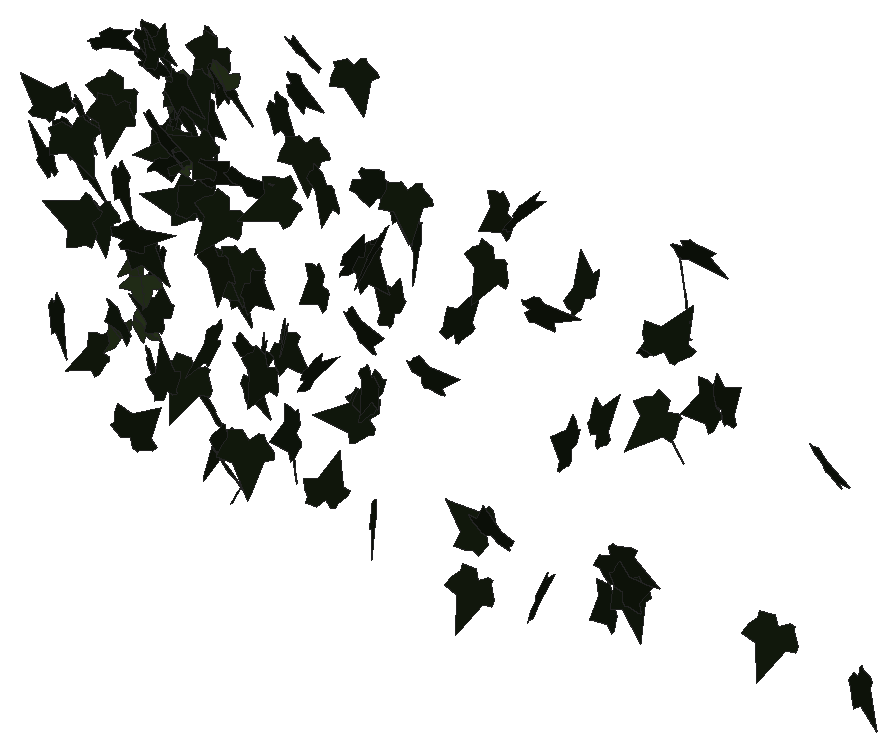
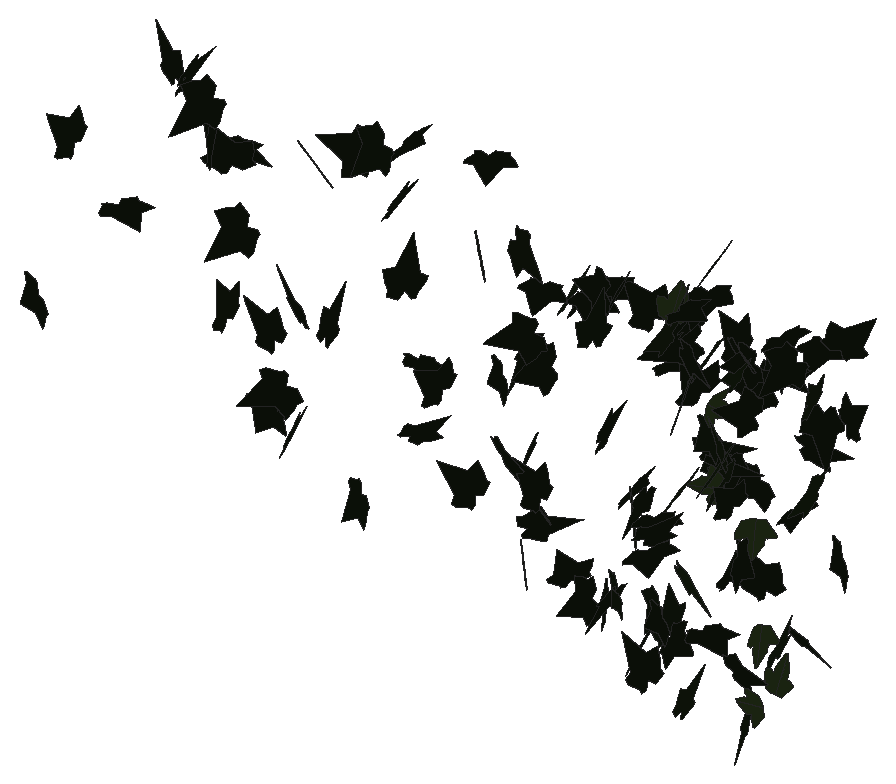
# SketchUp Ruby script. Lengths in inches.
U = 1.inch
M = Sketchup.active_model
def pt(a) = Geom::Point3d.new(a.map { |v| v * U })
def face(e, loops, mat)
  f = e.add_face(loops[0].map { |a| pt(a) })
  loops[1..].each { |l| e.add_face(l.map { |a| pt(a) }).erase! }
  f.material = f.back_material = mat if mat
  f
end
# faces: each face lists its corners as indices into pts; further lists are holes
def faces(e, pts, list, mat = nil) = list.each { |f| face(e, (f[0].is_a?(Array) ? f : [f]).map { |l| l.map { |i| pts[i] } }, mat) }
# xy, xz, yz: faces in a plane at the given z, y or x. An outline is a flat list of corners, or four numbers for a rectangle; further outlines are holes
def ring(l) = l.size == 4 ? [[l[0], l[1]], [l[2], l[1]], [l[2], l[3]], [l[0], l[3]]] : l.each_slice(2).to_a
def flat(e, list, mat, &to3) = list.each { |f| face(e, (f[0].is_a?(Array) ? f : [f]).map { |l| ring(l).map { |u, v| to3.(u, v) } }, mat) }
def xy(e, z, list, mat = nil) = flat(e, list, mat) { |x, y| [x, y, z] }
def xz(e, y, list, mat = nil) = flat(e, list, mat) { |x, z| [x, y, z] }
def yz(e, x, list, mat = nil) = flat(e, list, mat) { |y, z| [x, y, z] }
def lines(e, pts, list) = list.each { |a, b| e.add_line(pt(pts[a]), pt(pts[b])) }
# prism: a flat outline (further loops are holes) pulled along v
def prism(e, loops, v, mat = nil)
  f = face(e, loops, mat); d = Geom::Vector3d.new(v.map { |x| x * U })
  f.pushpull(f.normal.samedirection?(d) ? d.length : -d.length)
end
def box(e, o, s, mat = nil) = prism(e, [[o, [o[0] + s[0], o[1], o[2]], [o[0] + s[0], o[1] + s[1], o[2]], [o[0], o[1] + s[1], o[2]]]], [0, 0, s[2]], mat)
def at(x, y, z, deg = 0) = Geom::Transformation.translation(pt([x, y, z])) * Geom::Transformation.rotation(ORIGIN, Z_AXIS, deg.degrees)
def axes(o, x, y, z) = Geom::Transformation.new([*x, 0, *y, 0, *z, 0, *pt(o).to_a, 1])
def part(name) = M.definitions.add(name)
# library, detail: a bought-in or finely detailed component or shape, given as its bounding box
def library(name, o, s) = part(name).tap { |d| box(d.entities, o, s) }
def detail(e, o, s) = box(e.add_group.entities, o, s)
def put(e, d, t, mat = nil) = e.add_instance(d, t).tap { |i| i.material = mat if mat }
def group(e, t, mat = nil) = e.add_group.tap { |g| g.transformation = t; g.material = mat if mat }.entities
root = M.entities
M.materials.add("efeu1").color = [18, 25, 13]
M.materials.add("efeu2").color = [43, 57, 29]
c1 = part("ivyleaf_9")
p = [[1.54,2.16,1.25],[1.36,2.04,1.19],[-0.21,0.99,0.68],[-0.71,1.11,0.82],[-0.85,0.86,0.67],[-0.8,0.17,0.21],
  [-0.9,-0.01,0.1],[-0.67,-0.16,-0.02],[-0.08,-0.08,-0.05],[-0.03,-0.6,-0.4],[0.65,-0.88,-0.66],[0.83,-0.6,-0.49],
  [1.29,-0.42,-0.43],[1.8125,-0.07,-0.26],[1.21,0.44,0.15]]
faces(c1.entities,p,[[0,1,2,3,4,5,6,7,8,9,10,11,12,13,14]],"efeu1")
c2 = part("ivyleaf_10")
p = [[0,0.5,-0.03],[-0.0625,2.02,-0.43],[-0.19,2.01,-0.46],[-0.54,1.05,-0.29],[-0.52,0.625,-0.18],[-0.83,0.76,-0.28],
  [-1.16,0.64,-0.33],[-1.15,0.33,-0.24],[-0.77,-0.39,0.02],[-0.3,-0.51,0.16],[0.04,-0.48,0.23],[-0.02,2.01,-0.4375],
  [-0.06,2.01,-0.43],[0.04,-0.49,0.23],[0.67,-0.49,0.14],[1.38,0.36,-0.2],[1.375,0.51,-0.24],[0.81,0.65,-0.19],
  [0.62,0.59,-0.15],[0.6,1.09,-0.28],[0.5,1.23,-0.31]]
faces(c2.entities,p,[[0,1,2,3,4,5,6,7,8,9,10],[11,12,0,13,14,15,16,17,18,19,20]],"efeu2")
put(root,c1,axes([622.18,119.2,263.21],[1.07027,-0.87994,-0.07632],[-0.0577,0.04999,-1.38556],[0.88136,1.07182,0.00197]))
put(root,c2,axes([623.27,124.4375,252.77],[-0.24136,-1.16635,-0.4298],[0.08796,0.4207,-1.19106],[1.2399,-0.25688,0.00083]))
put(root,c1,axes([623.84,113.15,265.97],[0.21287,-0.39615,1.24207],[-0.67814,1.04122,0.44831],[-1.11347,-0.70987,-0.03558]))
put(root,c1,axes([623.82,116.15,267.9375],[0.91937,0.46952,-1.02129],[-0.91999,-0.44374,-1.03219],[-0.64582,1.30052,0.01652]))
put(root,c2,axes([623.56,122.17,247.09],[-0.30293,-0.92854,-0.79827],[-0.11742,-0.79652,0.97106],[-1.21887,0.30751,0.10485]))
put(root,c2,axes([623.04,125.3,246.88],[-0.31561,0.08385,-1.18043],[1.06121,-0.52059,-0.32072],[-0.5237,-1.10544,0.0615]))
put(root,c1,axes([623.75,119.875,274.29],[0.96359,0.79758,0.36569],[0.28178,0.23309,-1.25086],[-0.83094,1.00394,-0.00011]))
put(root,c1,axes([625.05,112.375,271.84],[0.34068,0.08173,1.27704],[-1.27575,0.12473,0.33236],[-0.09978,-1.3158,0.11083]))
put(root,c1,axes([624.23,121.375,249.1875],[0.80971,-0.82826,-0.57852],[0.44902,-0.36912,1.15692],[-0.90503,-0.92416,0.05641]))
put(root,c1,axes([624.83,124.15,244.65],[0.77824,-0.30414,-0.90228],[-0.84618,0.31337,-0.83549],[0.43656,1.14959,-0.01096]))
put(root,c1,axes([625.83,124.41,248.55],[-0.49007,0.3241,1.15418],[-0.93577,0.67596,-0.58715],[-0.74933,-1.05611,-0.02161]))
put(root,c1,axes([625.77,117.2,248.65],[-1.16585,0.35783,0.27903],[-0.26928,0.07359,-1.21949],[-0.36522,-1.19651,0.00844]))
put(root,c1,axes([624.35,116.86,269.05],[0.277,-0.84104,1.03036],[0.28803,-0.98956,-0.88517],[1.29847,0.39892,-0.02345]))
put(root,c1,axes([624.78,118.23,260.3],[0.0021,-1.203,-0.29037],[0.00436,0.29038,-1.20299],[1.23754,0.00102,0.00473]))
put(root,c1,axes([624.51,113.15,253.97],[-0.26944,-0.07175,-1.46481],[1.46634,-0.03975,-0.26777],[-0.02617,-1.48886,0.07774]))
put(root,c1,axes([625.69,124.93,263.3],[-0.31911,-0.34503,1.1605],[0.75283,0.88335,0.46964],[-0.94818,0.81748,-0.01768]))
put(root,c1,axes([624.77,123.65,270.93],[0.86711,-0.31452,0.89042],[0.83413,-0.31165,-0.92237],[0.44273,1.20316,-0.00615]))
put(root,c1,axes([625.96,125.93,267.32],[0.90464,-1.06864,-0.39949],[-0.25391,0.30847,-1.40012],[1.11226,0.93958,0.0053]))
put(root,c1,axes([627.81,113.16,262.51],[-0.88339,-0.44861,-1.11531],[-0.97594,-0.54051,0.99041],[-0.70192,1.31611,0.02659]))
put(root,c1,axes([627,117.99,271.59],[-1.15565,-0.89341,0.10894],[-0.06996,-0.0876,-1.46049],[0.89731,-1.15747,0.02644]))
put(root,c1,axes([625.91,122.21,274.46],[0.15475,0.02861,-1.2753],[1.15452,0.54319,0.15228],[0.54249,-1.16417,0.03971]))
put(root,c1,axes([628.12,121.07,273.8],[-0.28165,0.51474,1.17737],[-0.65843,0.97725,-0.58476],[-1.10347,-0.7145,0.04841]))
put(root,c1,axes([626.48,122.77,273.85],[0.77343,-0.98251,0.29118],[0.17618,-0.23187,-1.2504],[1.00949,0.79323,-0.00486]))
put(root,c1,axes([627.22,124.08,266.52],[-0.18666,0.93539,0.88445],[0.18438,-0.86506,0.95379],[1.27405,0.26223,-0.00846]))
put(root,c1,axes([627.3,111.75,271.08],[-0.23408,-0.97827,-1.00749],[0.26411,0.97249,-1.00565],[1.37923,-0.35225,0.02158]))
put(root,c1,axes([628.34,124.27,268.51],[-0.60417,0.68238,-1.01169],[-0.7456,0.68726,0.90882],[0.96605,0.95719,0.06871]))
put(root,c1,axes([627.82,122.83,265.22],[1.01108,-0.07908,-0.8091],[-0.75922,0.36981,-0.98489],[0.29066,1.24104,0.24192]))
put(root,c1,axes([628.98,122.97,264.77],[-0.92686,-0.02912,0.90525],[-0.89854,-0.13313,-0.92428],[0.11376,-1.28873,0.07503]))
put(root,c1,axes([628.17,121.08,256.2],[-0.35432,0.30629,-1.39728],[1.10967,-0.84953,-0.46761],[-0.90268,-1.16456,-0.02638]))
put(root,c1,axes([628.85,121.47,264.74],[0.40682,1.19247,-0.27089],[-0.08824,-0.25611,-1.25996],[-1.21967,0.41628,0.00081]))
put(root,c2,axes([628.59,123.68,270.375],[-0.11528,-0.76405,1.00801],[0.36573,-0.98909,-0.70788],[1.21083,0.22601,0.30978]))
put(root,c2,axes([628.01,123.84,263.55],[0.15172,-0.20456,1.22546],[1.15878,0.46861,-0.06525],[-0.44814,1.14245,0.24618]))
put(root,c1,axes([629.08,114.7,272.33],[-0.3971,-1.2906,-0.0785],[0.02506,0.07442,-1.35031],[1.29274,-0.39788,0.00207]))
put(root,c2,axes([629.93,116.92,256.45],[-0.99413,-0.79052,-0.06912],[0.05445,0.04258,-1.27013],[0.79167,-0.99562,0.00056]))
put(root,c1,axes([631.32,123.69,274.27],[-0.23925,-0.04646,-1.29065],[-1.27695,-0.18787,0.24347],[-0.19322,1.29913,-0.01094]))
put(root,c1,axes([630.01,116.37,260.27],[-0.13631,-0.21723,-1.44326],[1.28299,0.6732,-0.2225],[0.69579,-1.28389,0.12753]))
put(root,c1,axes([631.76,123.4375,242.82],[0.69343,-1.07414,0.27797],[-0.14309,0.23848,1.2785],[-1.10026,-0.70798,0.00892]))
put(root,c1,axes([632.78,119.19,263.15],[-0.60952,-0.00036,1.19221],[-1.18995,-0.08215,-0.60839],[0.07331,-1.33646,0.03708]))
put(root,c1,axes([631.26,126.67,252.28],[-0.18518,-0.11555,-1.22632],[1.21137,0.20757,-0.20248],[0.22314,-1.22273,0.08152]))
put(root,c1,axes([632.2,120.18,247.92],[-1.05369,-1.03255,-0.1616],[0.11127,0.11735,-1.47526],[1.03918,-1.05953,-0.0059]))
put(root,c1,axes([631.47,120.54,272.29],[0.80313,-1.25451,-0.12099],[-0.06212,0.10389,-1.48957],[1.2588,0.80552,0.00369]))
put(root,c1,axes([631.42,112.3,268.39],[-0.2568,-0.10479,-1.39468],[1.3967,0.05486,-0.26129],[0.07306,-1.41706,0.09302]))
put(root,c1,axes([632.64,121.67,269.87],[0.68175,-0.29692,-1.08173],[-0.92173,0.57315,-0.73824],[0.6393,1.14299,0.08918]))
put(root,c1,axes([632.33,115.8,270.74],[0.22031,-0.5165,1.38292],[0.83994,-1.10599,-0.54688],[1.21398,0.85895,0.12741]))
put(root,c1,axes([633.59,121.35,276.01],[-0.65952,-1.09232,0.3337],[-0.17864,-0.28195,-1.27596],[1.1281,-0.68324,-0.00696]))
put(root,c1,axes([634.04,114.76,249.52],[-0.44697,-0.88498,0.81564],[0.35961,0.73212,0.99142],[-1.14854,0.57363,-0.007]))
put(root,c1,axes([632.85,126.42,246.47],[-0.0673,-0.27756,1.4356],[1.06227,-0.99684,-0.14293],[1.00478,1.03528,0.24727]))
put(root,c1,axes([634.93,119.57,251.89],[-1.22281,0.66405,-0.36378],[0.30845,-0.19418,-1.3913],[-0.69149,-1.26091,0.02268]))
put(root,c1,axes([633.47,110.47,264.24],[0.59624,-0.00277,1.21045],[1.20694,0.10396,-0.59428],[-0.09204,1.34531,0.04842]))
put(root,c1,axes([633.86,110.71,247.08],[-0.49127,0.04059,1.4223],[1.23333,-0.7382,0.44707],[0.70956,1.31123,0.20766]))
put(root,c1,axes([634.4,117.12,275.39],[-0.22894,-1.17344,-0.9063],[0.14169,0.89553,-1.19529],[1.4759,-0.268,-0.02584]))
put(root,c1,axes([635.96,122.51,255.85],[-0.79796,-1.07819,-0.15225],[-0.05484,-0.14873,1.34063],[-1.08751,0.79862,0.04412]))
put(root,c1,axes([635.07,122.62,257.91],[-0.496,-1.10169,-0.50895],[0.25937,0.44088,-1.20712],[1.18553,-0.55738,0.05116]))
put(root,c2,axes([635.63,119.71,274.39],[-0.96165,-0.72892,-0.38434],[-0.29624,-0.24538,1.20658],[-0.76895,1.00612,0.01582]))
put(root,c1,axes([634.76,121.05,273.53],[1.01452,-0.84116,0.1064],[0.09072,-0.05727,-1.31781],[0.84299,1.01848,0.01377]))
put(root,c1,axes([634.92,119.95,258.86],[0.20491,-1.34864,0.64485],[0.13917,-0.63084,-1.36357],[1.48839,0.24466,0.03873]))
put(root,c1,axes([635.2,119.86,274.66],[0.17078,-0.82121,0.94718],[0.14708,-0.9362,-0.83821],[1.24495,0.22326,-0.03091]))
put(root,c1,axes([635.53,113.87,277.01],[0.88927,-0.64732,-0.83166],[-0.48519,0.71453,-1.07495],[0.93556,0.98585,0.23303]))
put(root,c1,axes([635.87,122.6,247.44],[0.79596,-0.77627,-0.72363],[-0.52901,0.49392,-1.11174],[0.91999,0.95563,-0.0132]))
put(root,c1,axes([636.26,115.63,265.55],[-0.5266,-0.48738,1.32358],[0.94978,0.92196,0.71737],[-1.04275,1.08589,-0.01501]))
put(root,c1,axes([636.92,118.26,244.9],[-0.17471,0.28734,-1.27841],[0.78194,-1.01203,-0.33433],[-1.0514,-0.8004,-0.03621]))
put(root,c1,axes([637.51,115.73,270.51],[-0.04019,-1.39427,-0.33401],[0.01694,-0.33458,1.39461],[-1.43362,0.03513,0.02584]))
put(root,c1,axes([638.36,123.11,250.39],[-0.08043,0.44334,1.26449],[-0.12729,1.25851,-0.44934],[-1.3339,-0.14683,-0.03337]))
put(root,c1,axes([637.8125,126.75,274.55],[1.17749,-0.62437,0.12941],[-0.10996,0.06886,1.33276],[-0.62809,-1.18258,0.00928]))
put(root,c1,axes([638.11,120.04,257.71],[0.43166,-0.46621,-1.10809],[-0.67274,0.88207,-0.63318],[0.99631,0.79759,0.05255]))
put(root,c1,axes([637.36,115.35,269.32],[1.17512,0.32103,0.82368],[0.80095,0.19327,-1.21801],[-0.37416,1.42197,-0.02041]))
put(root,c1,axes([638.19,123.79,250.8],[0.60817,-0.66893,-0.96136],[-0.45712,0.86175,-0.88881],[1.0783,0.74261,0.16543]))
put(root,c1,axes([639.64,115.19,266.71],[-0.79558,-1.14656,0.49012],[-0.22827,-0.43763,-1.39432],[1.22585,-0.82562,0.05844]))
put(root,c1,axes([638.94,115.86,244.03],[1.18805,-0.46251,-0.71038],[0.66346,-0.25392,1.2749],[-0.52761,-1.36075,0.00356]))
put(root,c1,axes([640.59,118.17,252.35],[-0.17886,0.60802,1.17923],[0.09386,-1.18111,0.62323],[1.32342,0.16594,0.11517]))
put(root,c1,axes([640.93,123.17,249.04],[0.30763,0.62151,1.16267],[0.52505,1.03738,-0.69346],[-1.2093,0.60851,-0.00531]))
put(root,c1,axes([641,119.45,274.53],[0.82976,-0.82381,-0.73705],[-0.55298,0.48863,-1.16869],[0.95714,0.99648,-0.03625]))
put(root,c1,axes([641.97,113.66,243.86],[0.02463,0.83925,1.01161],[0.02529,1.0113,-0.83961],[-1.31418,0.03519,0.00281]))
put(root,c1,axes([640.78,121.76,275.24],[0.53793,-0.026,-1.2387],[1.20426,0.32843,0.51608],[0.29126,-1.30992,0.15398]))
put(root,c1,axes([641.5625,114.74,269.83],[0.09338,-0.55313,1.27344],[1.18985,-0.62581,-0.35908],[0.71544,1.11298,0.43097]))
put(root,c1,axes([642.92,113.7,248.35],[-0.42401,-1.40267,-0.37145],[0.1509,0.34226,-1.4647],[1.44316,-0.4479,0.04401]))
put(root,c1,axes([643.21,115.38,254.23],[-0.17485,-1.21944,0.77996],[-0.10639,-0.77268,-1.2319],[1.44362,-0.20464,0.00369]))
put(root,c1,axes([642.82,118.96,246.3],[0.05367,-0.00351,-1.34428],[1.2969,-0.3539,0.0527],[-0.35376,-1.29797,-0.01074]))
put(root,c1,axes([643.88,125.35,276.29],[-0.5899,-0.77371,-0.86052],[0.518,0.68716,-0.97294],[1.0348,-0.78504,-0.00353]))
put(root,c1,axes([644.17,119.05,272.33],[-0.72218,-0.88228,-0.72869],[0.45476,0.56942,-1.14013],[1.05005,-0.8534,-0.00738]))
put(root,c1,axes([646.24,114.34,270.47],[-1.12452,-0.46434,0.75827],[-0.70168,-0.28743,-1.21661],[0.5461,-1.32548,-0.00181]))
put(root,c1,axes([646.7,122.29,255.63],[0.22077,-0.35198,1.40349],[0.9527,-1.03321,-0.40898],[1.08906,0.9752,0.07326]))
put(root,c1,axes([647.42,117.36,270.73],[0.1929,-1.20407,0.89151],[0.13731,-0.88088,-1.21942],[1.49189,0.23676,-0.00304]))
put(root,c1,axes([647.68,121.86,269.31],[0.19586,0.22557,-1.35132],[0.85718,1.04469,0.29862],[1.06873,-0.87923,0.00813]))
put(root,c1,axes([649.7,122.8,258.23],[-0.29766,0.50802,1.2762],[-0.77063,1.01919,-0.58545],[-1.13706,-0.82374,0.06271]))
put(root,c1,axes([648.87,115.62,244.78],[-0.7686,-0.37262,0.95698],[0.84838,0.44319,0.85395],[-0.5787,1.14461,-0.01911]))
put(root,c1,axes([649.97,119.29,250.41],[-0.64965,-0.15523,1.24591],[-1.1823,-0.39649,-0.66588],[0.42256,-1.34801,0.05238]))
put(root,c1,axes([648.375,124.75,266.67],[-0.19373,-0.06228,-1.29895],[1.29856,0.06138,-0.19661],[0.06996,-1.31189,0.05247]))
put(root,c1,axes([649.03,118.1,264.25],[0.33585,0.5858,1.30395],[0.60846,1.15347,-0.67492],[-1.29353,0.69468,0.02108]))
put(root,c1,axes([651.41,118.29,253.11],[-0.87162,0.87263,0.69734],[-0.49843,0.48775,-1.23335],[-0.99967,-1.00404,0.00693]))
put(root,c1,axes([650.7,109.61,253.68],[-0.14995,-0.40476,1.41284],[-0.37209,-1.36345,-0.4301],[1.42179,-0.39951,0.03644]))
put(root,c1,axes([651.03,117.85,265.4],[0.5261,-0.7021,-1.18884],[-0.75567,0.91834,-0.87675],[1.15553,0.92021,-0.03209]))
put(root,c1,axes([651.61,111.67,265.99],[-0.19305,-0.65064,1.1755],[-0.19411,-1.16161,-0.67482],[1.32946,-0.26408,0.07217]))
put(root,c1,axes([651.65,117.54,255.24],[0.38834,-0.25591,-1.24287],[0.98968,-0.75241,0.46416],[-0.7942,-1.06274,-0.02933]))
put(root,c1,axes([653.28,115.97,245.14],[-0.45224,0.10993,-1.24466],[1.20481,-0.31252,-0.46536],[-0.33122,-1.28687,0.00669]))
put(root,c1,axes([652.9375,122.45,253.77],[0.29844,-0.35075,1.32122],[1.16857,-0.63624,-0.43286],[0.7093,1.19579,0.15723]))
put(root,c1,axes([655.82,113.46,270.6875],[-0.8327,0.72894,-1.02479],[0.73937,-0.71045,-1.10613],[-1.01729,-1.11303,0.0349]))
put(root,c1,axes([657.68,120.45,260.3125],[-0.17635,-0.26448,1.37965],[0.88082,1.06237,0.31624],[-1.09433,0.89772,0.03222]))
put(root,c1,axes([657.51,116.12,270.8],[-0.65113,0.17954,-1.23752],[1.19697,-0.31427,-0.67539],[-0.36187,-1.36259,-0.00729]))
put(root,c1,axes([659.375,112.46,276.52],[-0.61602,-1.03523,-0.66624],[0.37333,0.55282,-1.20419],[1.17312,-0.71954,0.03337]))
put(root,c1,axes([663.73,118.93,273.35],[-0.33584,-0.6519,1.17848],[-0.24879,-1.16363,-0.71459],[1.32359,-0.38413,0.1647]))
put(root,c1,axes([666.94,112.31,249.45],[-0.85511,-0.99666,-0.29529],[-0.19267,-0.22378,1.31322],[-1.02148,0.87655,-0.0005]))
put(root,c1,axes([667.5,115.45,275.91],[0.39067,0.99458,1.02562],[0.30254,0.98157,-1.0671],[-1.39627,0.49097,0.05575]))
put(root,c1,axes([668.3,111.73,274.01],[-0.3489,-1.28927,0.65454],[-0.1239,-0.64419,-1.33493],[1.44059,-0.36766,0.04372]))
put(root,c1,axes([670.375,114.43,243.93],[-0.43358,0.64062,-1.22328],[-0.93936,0.80295,0.75345],[1.01213,1.01965,0.17523]))
put(root,c1,axes([672.52,104.46,250.58],[-1.25031,-0.62231,-0.41862],[0.37499,0.18608,-1.39662],[0.64954,-1.30533,0.00048]))
put(root,c1,axes([672.87,115.37,257.59],[0.08973,0.22298,1.4847],[-0.51122,-1.39393,0.24025],[1.41163,-0.51898,-0.00737]))
put(root,c1,axes([674.76,114.81,271.83],[-1.25751,0.45835,-0.70147],[-0.67146,0.2056,1.33804],[0.50129,1.42518,0.03257]))
put(root,c1,axes([672.76,111.06,271.54],[0.7855,0.53092,-1.0637],[0.887,0.58715,0.94807],[0.79156,-1.18479,-0.00682]))
put(root,c1,axes([674.58,103.68,255.84],[1.34706,-0.46156,0.34499],[-0.30054,0.18566,1.42191],[-0.49166,-1.37809,0.07601]))
put(root,c1,axes([674.57,116.62,259.12],[-0.52528,0.8642,1.07558],[0.54234,-0.92893,1.01123],[1.2687,0.7549,0.01305]))
put(root,c1,axes([677.57,114.43,245.99],[-0.15676,-0.55458,1.34874],[-0.14951,-1.34325,-0.5697],[1.45062,-0.19838,0.08703]))
put(root,c1,axes([677.76,119.29,266.85],[0.73633,1.00964,0.83519],[0.4544,0.70182,-1.24903],[-1.229,0.86439,0.03858]))
put(root,c1,axes([678.11,114.03,250.53],[-0.00917,0.07122,-1.46837],[0.90293,1.15906,0.05058],[1.16013,-0.90154,-0.05098]))
put(root,c1,axes([679.11,119.75,258.88],[0.18508,-0.69155,1.3362],[0.61091,-1.19576,-0.70348],[1.37494,0.62438,0.1327]))
put(root,c1,axes([679.66,114.23,248.33],[-0.72903,-0.404,-1.21646],[1.12326,0.47281,-0.8302],[0.61748,-1.33706,0.07399]))
put(root,c1,axes([682.42,117.84,271.52],[0.08727,-0.54139,1.41505],[-0.24665,1.39341,0.54832],[-1.49487,-0.26151,-0.00786]))
put(root,c1,axes([681.42,118.8,276.61],[1.46289,0.34522,0.16055],[0.15599,0.03799,-1.50307],[-0.3473,1.47118,0.00114]))
put(root,c1,axes([682.06,115.54,269.39],[-0.81305,-0.08015,1.26785],[1.26398,-0.20199,0.79779],[0.1274,1.49254,0.17605]))
put(root,c1,axes([682.78,109.55,251.18],[0.07669,-0.0126,1.4292],[1.0252,-0.99677,-0.0638],[0.99586,1.0271,-0.04438]))
put(root,c1,axes([685.99,110.61,267.39],[-1.28559,-0.62066,0.25406],[-0.21207,-0.14489,-1.42708],[0.63624,-1.30242,0.03768]))
put(root,c1,axes([691.55,109.53,270.47],[-0.35981,-0.41985,1.36113],[-0.45208,-1.29764,-0.51977],[1.35077,-0.54614,0.18862]))
put(root,c1,axes([692.63,109.3,270.75],[-0.31438,0.32855,1.40055],[0.72962,-1.19911,0.44508],[1.23981,0.78898,0.09322]))
put(root,c1,axes([698.08,114.83,265.34],[0.50924,-0.68949,1.23167],[0.83398,-0.90943,-0.85391],[1.13881,0.97431,0.07458]))
put(root,c1,axes([700.16,106.52,255.33],[-0.98896,-1.09487,-0.20165],[0.13905,0.14613,-1.47538],[1.10457,-0.99867,0.00519]))
put(root,c1,axes([703.18,112.76,249.18],[-0.22465,-0.18231,-1.48321],[1.48211,0.16459,-0.24471],[0.19107,-1.49107,0.15434]))
